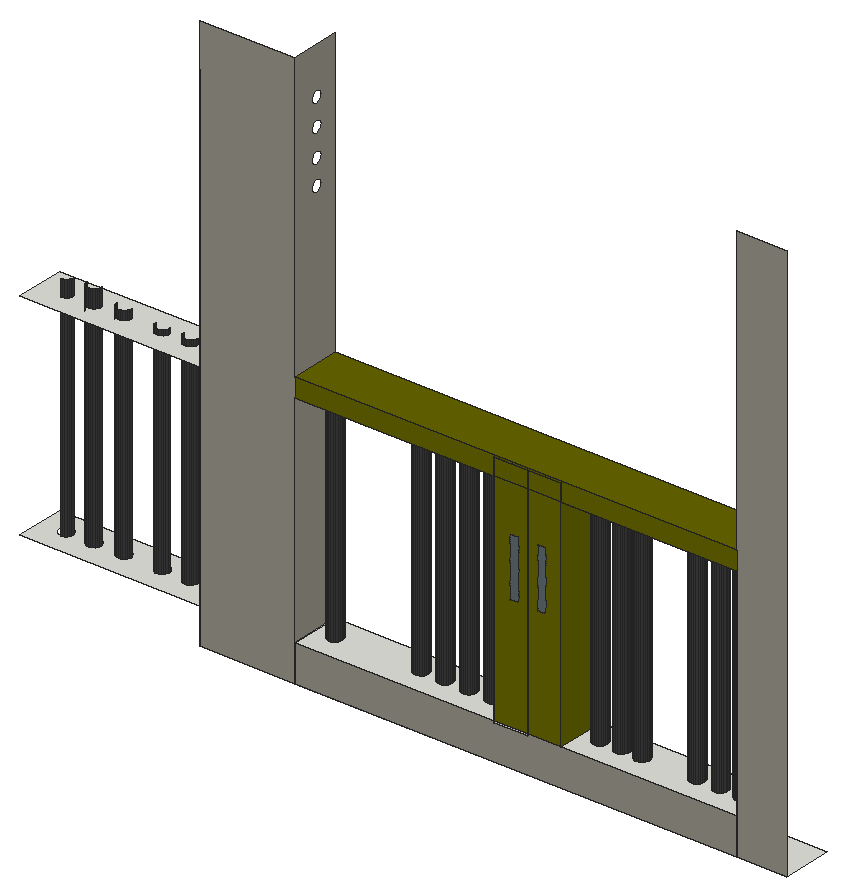
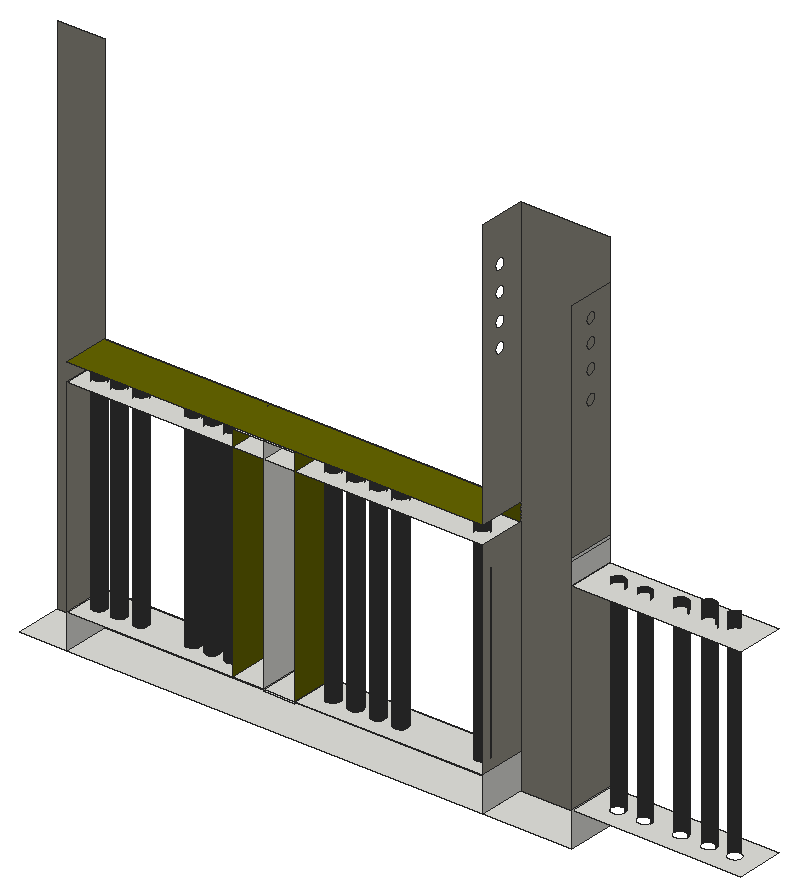
# SketchUp Ruby script. Lengths in inches.
U = 1.inch
M = Sketchup.active_model
def pt(a) = Geom::Point3d.new(a.map { |v| v * U })
def face(e, loops, mat)
  f = e.add_face(loops[0].map { |a| pt(a) })
  loops[1..].each { |l| e.add_face(l.map { |a| pt(a) }).erase! }
  f.material = f.back_material = mat if mat
  f
end
# faces: each face lists its corners as indices into pts; further lists are holes
def faces(e, pts, list, mat = nil) = list.each { |f| face(e, (f[0].is_a?(Array) ? f : [f]).map { |l| l.map { |i| pts[i] } }, mat) }
# xy, xz, yz: faces in a plane at the given z, y or x. An outline is a flat list of corners, or four numbers for a rectangle; further outlines are holes
def ring(l) = l.size == 4 ? [[l[0], l[1]], [l[2], l[1]], [l[2], l[3]], [l[0], l[3]]] : l.each_slice(2).to_a
def flat(e, list, mat, &to3) = list.each { |f| face(e, (f[0].is_a?(Array) ? f : [f]).map { |l| ring(l).map { |u, v| to3.(u, v) } }, mat) }
def xy(e, z, list, mat = nil) = flat(e, list, mat) { |x, y| [x, y, z] }
def xz(e, y, list, mat = nil) = flat(e, list, mat) { |x, z| [x, y, z] }
def yz(e, x, list, mat = nil) = flat(e, list, mat) { |y, z| [x, y, z] }
def lines(e, pts, list) = list.each { |a, b| e.add_line(pt(pts[a]), pt(pts[b])) }
# prism: a flat outline (further loops are holes) pulled along v
def prism(e, loops, v, mat = nil)
  f = face(e, loops, mat); d = Geom::Vector3d.new(v.map { |x| x * U })
  f.pushpull(f.normal.samedirection?(d) ? d.length : -d.length)
end
def box(e, o, s, mat = nil) = prism(e, [[o, [o[0] + s[0], o[1], o[2]], [o[0] + s[0], o[1] + s[1], o[2]], [o[0], o[1] + s[1], o[2]]]], [0, 0, s[2]], mat)
def at(x, y, z, deg = 0) = Geom::Transformation.translation(pt([x, y, z])) * Geom::Transformation.rotation(ORIGIN, Z_AXIS, deg.degrees)
def axes(o, x, y, z) = Geom::Transformation.new([*x, 0, *y, 0, *z, 0, *pt(o).to_a, 1])
def part(name) = M.definitions.add(name)
# library, detail: a bought-in or finely detailed component or shape, given as its bounding box
def library(name, o, s) = part(name).tap { |d| box(d.entities, o, s) }
def detail(e, o, s) = box(e.add_group.entities, o, s)
def put(e, d, t, mat = nil) = e.add_instance(d, t).tap { |i| i.material = mat if mat }
def group(e, t, mat = nil) = e.add_group.tap { |g| g.transformation = t; g.material = mat if mat }.entities
root = M.entities
M.materials.add("[Color E08]").color = [102, 102, 0]
M.materials.add("[Color M07]").color = [58, 58, 58]
M.materials.add("[Formica Graystone]").color = [149, 146, 135]
M.materials.add("[Formica Speckled Grey]").color = [94, 105, 111]
xy(root,0,[[82.62,52.46,91.56,57.16],[91.56,52.46,133.09,57.16],[133.09,52.46,137.78,57.16]])
xy(root,3.25,[[110.32,52.46,113.44,57.16]])
xy(root,3.4375,[[[65.76,52.46,82.62,57.16],[68.11,54.27,67.9375,54.29,67.77,54.36,67.63,54.47,67.52,54.61,67.45,54.78,67.43,54.96,67.45,55.13,67.52,55.3,67.63,55.44,67.77,55.55,67.9375,55.62,68.11,55.64,68.29,55.62,68.46,55.55,68.6,55.44,68.71,55.3,68.78,55.13,68.8,54.96,68.78,54.78,68.71,54.61,68.6,54.47,68.46,54.36,68.29,54.29],[79.8,54.27,79.625,54.29,79.46,54.36,79.32,54.47,79.21,54.61,79.14,54.78,79.11,54.96,79.14,55.13,79.21,55.3,79.32,55.44,79.46,55.55,79.625,55.62,79.8,55.64,79.98,55.62,80.15,55.55,80.29,55.44,80.4,55.3,80.47,55.13,80.49,54.96,80.47,54.78,80.4,54.61,80.29,54.47,80.15,54.36,79.98,54.29],[70.74,54.27,70.5625,54.29,70.4,54.36,70.25,54.47,70.14,54.61,70.07,54.78,70.05,54.96,70.07,55.13,70.14,55.3,70.25,55.44,70.4,55.55,70.5625,55.62,70.74,55.64,70.92,55.62,71.08,55.55,71.23,55.44,71.33,55.3,71.4,55.13,71.43,54.96,71.4,54.78,71.33,54.61,71.23,54.47,71.08,54.36,70.92,54.29],[77.18,54.27,77,54.29,76.83,54.36,76.69,54.47,76.58,54.61,76.51,54.78,76.49,54.96,76.51,55.13,76.58,55.3,76.69,55.44,76.83,55.55,77,55.62,77.18,55.64,77.35,55.62,77.52,55.55,77.66,55.44,77.77,55.3,77.84,55.13,77.86,54.96,77.84,54.78,77.77,54.61,77.66,54.47,77.52,54.36,77.35,54.29],[73.55,54.27,73.375,54.29,73.21,54.36,73.07,54.47,72.96,54.61,72.89,54.78,72.86,54.96,72.89,55.13,72.96,55.3,73.07,55.44,73.21,55.55,73.375,55.62,73.55,55.64,73.73,55.62,73.9,55.55,74.04,55.44,74.15,55.3,74.22,55.13,74.24,54.96,74.22,54.78,74.15,54.61,74.04,54.47,73.9,54.36,73.73,54.29]],[91.56,52.46,110.32,57.16],[110.32,52.46,113.44,57.16],[113.44,52.46,116.56,57.16],[116.56,52.46,133.09,57.16]])
xy(root,23.55,[[65.76,52.46,82.62,57.16]])
xy(root,24.05,[[91.56,52.46,133.09,57.16]])
xy(root,25.6875,[[110.32,52.46,113.44,57.16],[113.44,52.46,116.56,57.16]])
xy(root,25.83,[[91.56,52.46,133.09,57.16]],"[Color E08]")
xz(root,52.46,[[110.32,3.25,113.44,3.4375]])
xz(root,52.46,[[[110.32,3.4375,113.44,24.05],[111.77,14.14,112.58,19.7]],[[113.44,3.4375,116.56,24.05],[114.39,14.14,115.2,19.7]],[91.56,24.05,110.32,24.05,110.32,25.6875,116.56,25.6875,116.56,24.05,133.09,24.05,133.09,25.83,91.56,25.83],[110.32,24.05,113.44,25.6875],[113.44,24.05,116.56,25.6875]],"[Color E08]")
xz(root,52.46,[[82.62,0,91.56,52.6875],[91.56,0,133.09,0,133.09,3.4375,113.44,3.4375,113.44,3.25,110.32,3.25,110.32,3.4375,91.56,3.4375],[133.09,0,137.78,52.6875]],"[Formica Graystone]")
xz(root,52.46,[[111.77,14.14,112.58,19.7],[114.39,14.14,115.2,19.7]],"[Formica Speckled Grey]")
yz(root,82.62,[[52.46,0,57.16,3.4375],[52.46,23.55,57.16,25.6875],[52.46,25.6875,57.16,26.02]])
yz(root,82.62,[[52.46,3.4375,57.16,23.55],[[52.46,26.02,57.16,48.59],[54.84,38.61,54.99,38.63,55.12,38.68,55.24,38.77,55.33,38.89,55.38,39.03,55.4,39.17,55.38,39.32,55.33,39.45,55.24,39.57,55.12,39.66,54.99,39.72,54.84,39.73,54.69,39.72,54.56,39.66,54.44,39.57,54.35,39.45,54.3,39.32,54.28,39.17,54.3,39.03,54.35,38.89,54.44,38.77,54.56,38.68,54.69,38.63],[54.84,41.36,54.99,41.38,55.12,41.43,55.24,41.52,55.33,41.64,55.38,41.78,55.4,41.92,55.38,42.07,55.33,42.2,55.24,42.32,55.12,42.41,54.99,42.47,54.84,42.48,54.69,42.47,54.56,42.41,54.44,42.32,54.35,42.2,54.3,42.07,54.28,41.92,54.3,41.78,54.35,41.64,54.44,41.52,54.56,41.43,54.69,41.38],[54.84,43.67,54.99,43.69,55.12,43.75,55.24,43.84,55.33,43.95,55.38,44.09,55.4,44.23,55.38,44.38,55.33,44.52,55.24,44.63,55.12,44.72,54.99,44.78,54.84,44.8,54.69,44.78,54.56,44.72,54.44,44.63,54.35,44.52,54.3,44.38,54.28,44.23,54.3,44.09,54.35,43.95,54.44,43.84,54.56,43.75,54.69,43.69],[54.84,45.92,54.99,45.94,55.12,46,55.24,46.09,55.33,46.2,55.38,46.34,55.4,46.48,55.38,46.63,55.33,46.77,55.24,46.88,55.12,46.97,54.99,47.03,54.84,47.05,54.69,47.03,54.56,46.97,54.44,46.88,54.35,46.77,54.3,46.63,54.28,46.48,54.3,46.34,54.35,46.2,54.44,46.09,54.56,46,54.69,45.94]]],"[Formica Graystone]")
yz(root,91.56,[[52.46,0,57.16,3.4375]])
yz(root,91.56,[[52.46,3.4375,57.16,24.05],[[52.46,25.83,57.16,52.6875],[55.04,40.18,54.9,40.2,54.76,40.26,54.64,40.35,54.55,40.46,54.5,40.6,54.48,40.75,54.5,40.89,54.55,41.03,54.64,41.14,54.76,41.23,54.9,41.29,55.04,41.31,55.1875,41.29,55.32,41.23,55.4375,41.14,55.53,41.03,55.58,40.89,55.6,40.75,55.58,40.6,55.53,40.46,55.4375,40.35,55.32,40.26,55.1875,40.2],[55.04,47.68,54.9,47.7,54.76,47.76,54.64,47.85,54.55,47.96,54.5,48.1,54.48,48.25,54.5,48.39,54.55,48.53,54.64,48.64,54.76,48.73,54.9,48.79,55.04,48.81,55.1875,48.79,55.32,48.73,55.4375,48.64,55.53,48.53,55.58,48.39,55.6,48.25,55.58,48.1,55.53,47.96,55.4375,47.85,55.32,47.76,55.1875,47.7],[55.04,45.18,54.9,45.2,54.76,45.26,54.64,45.35,54.55,45.46,54.5,45.6,54.48,45.75,54.5,45.89,54.55,46.03,54.64,46.14,54.76,46.23,54.9,46.29,55.04,46.31,55.1875,46.29,55.32,46.23,55.4375,46.14,55.53,46.03,55.58,45.89,55.6,45.75,55.58,45.6,55.53,45.46,55.4375,45.35,55.32,45.26,55.1875,45.2],[55.04,42.56,54.9,42.58,54.76,42.63,54.64,42.72,54.55,42.84,54.5,42.98,54.48,43.12,54.5,43.27,54.55,43.4,54.64,43.52,54.76,43.61,54.9,43.66,55.04,43.68,55.1875,43.66,55.32,43.61,55.4375,43.52,55.53,43.4,55.58,43.27,55.6,43.12,55.58,42.98,55.53,42.84,55.4375,42.72,55.32,42.63,55.1875,42.58]]],"[Formica Graystone]")
yz(root,110.32,[[52.46,3.25,57.16,3.4375]])
yz(root,110.32,[[52.46,3.4375,57.16,25.6875]],"[Color E08]")
yz(root,113.44,[[52.46,3.25,57.16,3.4375],[52.46,3.4375,57.16,25.6875]])
yz(root,116.56,[[52.46,3.4375,57.16,25.6875]],"[Color E08]")
yz(root,133.09,[[52.46,0,57.16,3.4375]])
yz(root,133.09,[[52.46,3.4375,57.16,24.05]],"[Formica Graystone]")
p = [[68.11,54.27,3.4375],[68.29,54.29,3.4375],[68.29,54.29,25.0625],[68.11,54.27,25.0625],[68.46,54.36,3.4375],[68.46,54.36,25.0625],
  [70.4,54.36,3.4375],[70.5625,54.29,3.4375],[70.5625,54.29,25.1875],[70.4,54.36,25.1875],[70.74,54.27,3.4375],[70.74,54.27,25.1875],
  [70.92,54.29,3.4375],[70.92,54.29,25.1875],[71.08,54.36,3.4375],[71.08,54.36,25.1875],[73.21,54.36,3.4375],[73.375,54.29,3.4375],
  [73.375,54.29,24.375],[73.21,54.36,24.375],[73.55,54.27,3.4375],[73.55,54.27,24.375],[73.73,54.29,3.4375],[73.73,54.29,24.375],
  [73.9,54.36,3.4375],[73.9,54.36,24.375],[76.83,54.36,3.4375],[77,54.29,3.4375],[77,54.29,24],[76.83,54.36,24],
  [77.18,54.27,3.4375],[77.18,54.27,24],[77.35,54.29,3.4375],[77.35,54.29,24],[77.52,54.36,3.4375],[77.52,54.36,24],
  [79.46,54.36,3.4375],[79.625,54.29,3.4375],[79.625,54.29,24.0625],[79.46,54.36,24.0625],[79.8,54.27,3.4375],[79.8,54.27,24.0625],
  [79.98,54.29,3.4375],[79.98,54.29,24.0625],[80.15,54.36,3.4375],[80.15,54.36,24.0625],[93.02,54.36,3.4375],[93.1875,54.29,3.4375],
  [93.1875,54.29,25.1875],[93.02,54.36,25.1875],[93.36,54.27,3.4375],[93.36,54.27,25.1875],[93.54,54.29,3.4375],[93.54,54.29,25.1875],
  [93.71,54.36,3.4375],[93.71,54.36,25.1875],[101.15,54.36,3.4375],[101.3125,54.29,3.4375],[101.3125,54.29,25.1875],[101.15,54.36,25.1875],
  [101.49,54.27,3.4375],[101.49,54.27,25.1875],[101.67,54.29,3.4375],[101.67,54.29,25.1875],[101.83,54.36,3.4375],[101.83,54.36,25.1875],
  [103.4,54.36,3.4375],[103.5625,54.29,3.4375],[103.5625,54.29,25.1875],[103.4,54.36,25.1875],[103.74,54.27,3.4375],[103.74,54.27,25.1875],
  [103.92,54.29,3.4375],[103.92,54.29,25.1875],[104.08,54.36,3.4375],[104.08,54.36,25.1875],[105.65,54.36,3.4375],[105.8125,54.29,3.4375],
  [105.8125,54.29,25.1875],[105.65,54.36,25.1875],[105.99,54.27,3.4375],[105.99,54.27,25.1875],[106.17,54.29,3.4375],[106.17,54.29,25.1875],
  [106.33,54.36,3.4375],[106.33,54.36,25.1875],[107.9,54.36,3.4375],[108.0625,54.29,3.4375],[108.0625,54.29,25.1875],[107.9,54.36,25.1875],
  [108.24,54.27,3.4375],[108.24,54.27,25.1875],[108.42,54.29,3.4375],[108.42,54.29,25.1875],[108.58,54.36,3.4375],[108.58,54.36,25.1875],
  [117.96,54.36,3.4375],[118.125,54.29,3.4375],[118.125,54.29,25.1875],[117.96,54.36,25.1875],[118.3,54.27,3.4375],[118.3,54.27,25.1875],
  [118.48,54.29,3.4375],[118.48,54.29,25.1875],[118.65,54.36,3.4375],[118.65,54.36,25.1875],[119.96,54.36,3.4375],[120.125,54.29,3.4375],
  [120.125,54.29,25.1875],[119.96,54.36,25.1875],[120.3,54.27,3.4375],[120.3,54.27,25.1875],[120.48,54.29,3.4375],[120.48,54.29,25.1875],
  [120.65,54.36,3.4375],[120.65,54.36,25.1875],[121.9,54.36,3.4375],[122.0625,54.29,3.4375],[122.0625,54.29,25.1875],[121.9,54.36,25.1875],
  [122.24,54.27,3.4375],[122.24,54.27,25.1875],[122.42,54.29,3.4375],[122.42,54.29,25.1875],[122.58,54.36,3.4375],[122.58,54.36,25.1875],
  [127.08,54.36,3.4375],[127.25,54.29,3.4375],[127.25,54.29,25.1875],[127.08,54.36,25.1875],[127.43,54.27,3.4375],[127.43,54.27,25.1875],
  [127.6,54.29,3.4375],[127.6,54.29,25.1875],[127.77,54.36,3.4375],[127.77,54.36,25.1875],[129.27,54.36,3.4375],[129.4375,54.29,3.4375],
  [129.4375,54.29,25.1875],[129.27,54.36,25.1875],[129.61,54.27,3.4375],[129.61,54.27,25.1875],[129.79,54.29,3.4375],[129.79,54.29,25.1875],
  [129.96,54.36,3.4375],[129.96,54.36,25.1875],[131.27,54.36,3.4375],[131.4375,54.29,3.4375],[131.4375,54.29,25.1875],[131.27,54.36,25.1875],
  [131.61,54.27,3.4375],[131.61,54.27,25.1875],[131.79,54.29,3.4375],[131.79,54.29,25.1875],[131.96,54.36,3.4375],[131.96,54.36,25.1875],
  [68.6,54.47,3.4375],[68.6,54.47,25.0625],[70.25,54.47,3.4375],[70.25,54.47,25.1875],[71.23,54.47,3.4375],[71.23,54.47,25.1875],
  [73.07,54.47,3.4375],[73.07,54.47,24.375],[74.04,54.47,3.4375],[74.04,54.47,24.375],[76.69,54.47,3.4375],[76.69,54.47,24],
  [77.66,54.47,3.4375],[77.66,54.47,24],[79.32,54.47,3.4375],[79.32,54.47,24.0625],[80.29,54.47,3.4375],[80.29,54.47,24.0625],
  [92.88,54.47,3.4375],[92.88,54.47,25.1875],[93.85,54.47,3.4375],[93.85,54.47,25.1875],[101,54.47,3.4375],[101,54.47,25.1875],
  [101.98,54.47,3.4375],[101.98,54.47,25.1875],[103.25,54.47,3.4375],[103.25,54.47,25.1875],[104.23,54.47,3.4375],[104.23,54.47,25.1875],
  [105.5,54.47,3.4375],[105.5,54.47,25.1875],[106.48,54.47,3.4375],[106.48,54.47,25.1875],[107.75,54.47,3.4375],[107.75,54.47,25.1875],
  [108.73,54.47,3.4375],[108.73,54.47,25.1875],[117.82,54.47,3.4375],[117.82,54.47,25.1875],[118.79,54.47,3.4375],[118.79,54.47,25.1875],
  [119.82,54.47,3.4375],[119.82,54.47,25.1875],[120.79,54.47,3.4375],[120.79,54.47,25.1875],[121.75,54.47,3.4375],[121.75,54.47,25.1875],
  [122.73,54.47,3.4375],[122.73,54.47,25.1875],[126.94,54.47,3.4375],[126.94,54.47,25.1875],[127.91,54.47,3.4375],[127.91,54.47,25.1875],
  [129.13,54.47,3.4375],[129.13,54.47,25.1875],[130.1,54.47,3.4375],[130.1,54.47,25.1875],[131.13,54.47,3.4375],[131.13,54.47,25.1875],
  [132.1,54.47,3.4375],[132.1,54.47,25.1875],[68.71,54.61,3.4375],[68.71,54.61,25.0625],[70.14,54.61,3.4375],[70.14,54.61,25.1875],
  [71.33,54.61,3.4375],[71.33,54.61,25.1875],[72.96,54.61,3.4375],[72.96,54.61,24.375],[74.15,54.61,3.4375],[74.15,54.61,24.375],
  [76.58,54.61,3.4375],[76.58,54.61,24],[77.77,54.61,3.4375],[77.77,54.61,24],[79.21,54.61,3.4375],[79.21,54.61,24.0625],
  [80.4,54.61,3.4375],[80.4,54.61,24.0625],[92.77,54.61,3.4375],[92.77,54.61,25.1875],[93.96,54.61,3.4375],[93.96,54.61,25.1875],
  [100.89,54.61,3.4375],[100.89,54.61,25.1875],[102.08,54.61,3.4375],[102.08,54.61,25.1875],[103.14,54.61,3.4375],[103.14,54.61,25.1875],
  [104.33,54.61,3.4375],[104.33,54.61,25.1875],[105.39,54.61,3.4375],[105.39,54.61,25.1875],[106.58,54.61,3.4375],[106.58,54.61,25.1875],
  [107.64,54.61,3.4375],[107.64,54.61,25.1875],[108.83,54.61,3.4375],[108.83,54.61,25.1875],[117.71,54.61,3.4375],[117.71,54.61,25.1875],
  [118.9,54.61,3.4375],[118.9,54.61,25.1875],[119.71,54.61,3.4375],[119.71,54.61,25.1875],[120.9,54.61,3.4375],[120.9,54.61,25.1875],
  [121.64,54.61,3.4375],[121.64,54.61,25.1875],[122.83,54.61,3.4375],[122.83,54.61,25.1875],[126.83,54.61,3.4375],[126.83,54.61,25.1875],
  [128.02,54.61,3.4375],[128.02,54.61,25.1875],[129.02,54.61,3.4375],[129.02,54.61,25.1875],[130.21,54.61,3.4375],[130.21,54.61,25.1875],
  [131.02,54.61,3.4375],[131.02,54.61,25.1875],[132.21,54.61,3.4375],[132.21,54.61,25.1875],[68.78,54.78,3.4375],[68.78,54.78,25.0625],
  [70.07,54.78,3.4375],[70.07,54.78,25.1875],[71.4,54.78,3.4375],[71.4,54.78,25.1875],[72.89,54.78,3.4375],[72.89,54.78,24.375],
  [74.22,54.78,3.4375],[74.22,54.78,24.375],[76.51,54.78,3.4375],[76.51,54.78,24],[77.84,54.78,3.4375],[77.84,54.78,24],
  [79.14,54.78,3.4375],[79.14,54.78,24.0625],[80.47,54.78,3.4375],[80.47,54.78,24.0625],[92.7,54.78,3.4375],[92.7,54.78,25.1875],
  [94.03,54.78,3.4375],[94.03,54.78,25.1875],[100.82,54.78,3.4375],[100.82,54.78,25.1875],[102.15,54.78,3.4375],[102.15,54.78,25.1875],
  [103.07,54.78,3.4375],[103.07,54.78,25.1875],[104.4,54.78,3.4375],[104.4,54.78,25.1875],[105.32,54.78,3.4375],[105.32,54.78,25.1875],
  [106.65,54.78,3.4375],[106.65,54.78,25.1875],[107.57,54.78,3.4375],[107.57,54.78,25.1875],[108.9,54.78,3.4375],[108.9,54.78,25.1875],
  [117.64,54.78,3.4375],[117.64,54.78,25.1875],[118.97,54.78,3.4375],[118.97,54.78,25.1875],[119.64,54.78,3.4375],[119.64,54.78,25.1875],
  [120.97,54.78,3.4375],[120.97,54.78,25.1875],[121.57,54.78,3.4375],[121.57,54.78,25.1875],[122.9,54.78,3.4375],[122.9,54.78,25.1875],
  [126.76,54.78,3.4375],[126.76,54.78,25.1875],[128.09,54.78,3.4375],[128.09,54.78,25.1875],[128.95,54.78,3.4375],[128.95,54.78,25.1875],
  [130.28,54.78,3.4375],[130.28,54.78,25.1875],[130.95,54.78,3.4375],[130.95,54.78,25.1875],[132.28,54.78,3.4375],[132.28,54.78,25.1875],
  [68.8,54.96,3.4375],[68.8,54.96,25.0625],[70.05,54.96,3.4375],[70.05,54.96,25.1875],[71.43,54.96,3.4375],[71.43,54.96,25.1875],
  [72.86,54.96,3.4375],[72.86,54.96,24.375],[74.24,54.96,3.4375],[74.24,54.96,24.375],[76.49,54.96,3.4375],[76.49,54.96,24],
  [77.86,54.96,3.4375],[77.86,54.96,24],[79.11,54.96,3.4375],[79.11,54.96,24.0625],[80.49,54.96,3.4375],[80.49,54.96,24.0625],
  [92.68,54.96,3.4375],[92.68,54.96,25.1875],[94.05,54.96,3.4375],[94.05,54.96,25.1875],[100.8,54.96,3.4375],[100.8,54.96,25.1875],
  [102.18,54.96,3.4375],[102.18,54.96,25.1875],[103.05,54.96,3.4375],[103.05,54.96,25.1875],[104.43,54.96,3.4375],[104.43,54.96,25.1875],
  [105.3,54.96,3.4375],[105.3,54.96,25.1875],[106.68,54.96,3.4375],[106.68,54.96,25.1875],[107.55,54.96,3.4375],[107.55,54.96,25.1875],
  [108.93,54.96,3.4375],[108.93,54.96,25.1875],[117.61,54.96,3.4375],[117.61,54.96,25.1875],[118.99,54.96,3.4375],[118.99,54.96,25.1875],
  [119.61,54.96,3.4375],[119.61,54.96,25.1875],[120.99,54.96,3.4375],[120.99,54.96,25.1875],[121.55,54.96,3.4375],[121.55,54.96,25.1875],
  [122.93,54.96,3.4375],[122.93,54.96,25.1875],[126.74,54.96,3.4375],[126.74,54.96,25.1875],[128.11,54.96,3.4375],[128.11,54.96,25.1875],
  [128.93,54.96,3.4375],[128.93,54.96,25.1875],[130.3,54.96,3.4375],[130.3,54.96,25.1875],[130.93,54.96,3.4375],[130.93,54.96,25.1875],
  [132.3,54.96,3.4375],[132.3,54.96,25.1875],[92.7,55.13,3.4375],[92.7,55.13,25.1875],[94.03,55.13,3.4375],[94.03,55.13,25.1875],
  [100.82,55.13,3.4375],[100.82,55.13,25.1875],[102.15,55.13,3.4375],[102.15,55.13,25.1875],[103.07,55.13,3.4375],[103.07,55.13,25.1875],
  [104.4,55.13,3.4375],[104.4,55.13,25.1875],[105.32,55.13,3.4375],[105.32,55.13,25.1875],[106.65,55.13,3.4375],[106.65,55.13,25.1875],
  [107.57,55.13,3.4375],[107.57,55.13,25.1875],[108.9,55.13,3.4375],[108.9,55.13,25.1875],[117.64,55.13,3.4375],[117.64,55.13,25.1875],
  [118.97,55.13,3.4375],[118.97,55.13,25.1875],[119.64,55.13,3.4375],[119.64,55.13,25.1875],[120.97,55.13,3.4375],[120.97,55.13,25.1875],
  [121.57,55.13,3.4375],[121.57,55.13,25.1875],[122.9,55.13,3.4375],[122.9,55.13,25.1875],[126.76,55.13,3.4375],[126.76,55.13,25.1875],
  [128.09,55.13,3.4375],[128.09,55.13,25.1875],[128.95,55.13,3.4375],[128.95,55.13,25.1875],[130.28,55.13,3.4375],[130.28,55.13,25.1875],
  [130.95,55.13,3.4375],[130.95,55.13,25.1875],[132.28,55.13,3.4375],[132.28,55.13,25.1875],[92.77,55.3,3.4375],[92.77,55.3,25.1875],
  [93.96,55.3,3.4375],[93.96,55.3,25.1875],[100.89,55.3,3.4375],[100.89,55.3,25.1875],[102.08,55.3,3.4375],[102.08,55.3,25.1875],
  [103.14,55.3,3.4375],[103.14,55.3,25.1875],[104.33,55.3,3.4375],[104.33,55.3,25.1875],[105.39,55.3,3.4375],[105.39,55.3,25.1875],
  [106.58,55.3,3.4375],[106.58,55.3,25.1875],[107.64,55.3,3.4375],[107.64,55.3,25.1875],[108.83,55.3,3.4375],[108.83,55.3,25.1875],
  [117.71,55.3,3.4375],[117.71,55.3,25.1875],[118.9,55.3,3.4375],[118.9,55.3,25.1875],[119.71,55.3,3.4375],[119.71,55.3,25.1875],
  [120.9,55.3,3.4375],[120.9,55.3,25.1875],[121.64,55.3,3.4375],[121.64,55.3,25.1875],[122.83,55.3,3.4375],[122.83,55.3,25.1875],
  [126.83,55.3,3.4375],[126.83,55.3,25.1875],[128.02,55.3,3.4375],[128.02,55.3,25.1875],[129.02,55.3,3.4375],[129.02,55.3,25.1875],
  [130.21,55.3,3.4375],[130.21,55.3,25.1875],[131.02,55.3,3.4375],[131.02,55.3,25.1875],[132.21,55.3,3.4375],[132.21,55.3,25.1875],
  [92.88,55.44,3.4375],[92.88,55.44,25.1875],[93.85,55.44,3.4375],[93.85,55.44,25.1875],[101,55.44,3.4375],[101,55.44,25.1875],
  [101.98,55.44,3.4375],[101.98,55.44,25.1875],[103.25,55.44,3.4375],[103.25,55.44,25.1875],[104.23,55.44,3.4375],[104.23,55.44,25.1875],
  [105.5,55.44,3.4375],[105.5,55.44,25.1875],[106.48,55.44,3.4375],[106.48,55.44,25.1875],[107.75,55.44,3.4375],[107.75,55.44,25.1875],
  [108.73,55.44,3.4375],[108.73,55.44,25.1875],[117.82,55.44,3.4375],[117.82,55.44,25.1875],[118.79,55.44,3.4375],[118.79,55.44,25.1875],
  [119.82,55.44,3.4375],[119.82,55.44,25.1875],[120.79,55.44,3.4375],[120.79,55.44,25.1875],[121.75,55.44,3.4375],[121.75,55.44,25.1875],
  [122.73,55.44,3.4375],[122.73,55.44,25.1875],[126.94,55.44,3.4375],[126.94,55.44,25.1875],[127.91,55.44,3.4375],[127.91,55.44,25.1875],
  [129.13,55.44,3.4375],[129.13,55.44,25.1875],[130.1,55.44,3.4375],[130.1,55.44,25.1875],[131.13,55.44,3.4375],[131.13,55.44,25.1875],
  [132.1,55.44,3.4375],[132.1,55.44,25.1875],[93.02,55.55,3.4375],[93.02,55.55,25.1875],[93.71,55.55,3.4375],[93.71,55.55,25.1875],
  [101.15,55.55,3.4375],[101.15,55.55,25.1875],[101.83,55.55,3.4375],[101.83,55.55,25.1875],[103.4,55.55,3.4375],[103.4,55.55,25.1875],
  [104.08,55.55,3.4375],[104.08,55.55,25.1875],[105.65,55.55,3.4375],[105.65,55.55,25.1875],[106.33,55.55,3.4375],[106.33,55.55,25.1875],
  [107.9,55.55,3.4375],[107.9,55.55,25.1875],[108.58,55.55,3.4375],[108.58,55.55,25.1875],[117.96,55.55,3.4375],[117.96,55.55,25.1875],
  [118.65,55.55,3.4375],[118.65,55.55,25.1875],[119.96,55.55,3.4375],[119.96,55.55,25.1875],[120.65,55.55,3.4375],[120.65,55.55,25.1875],
  [121.9,55.55,3.4375],[121.9,55.55,25.1875],[122.58,55.55,3.4375],[122.58,55.55,25.1875],[127.08,55.55,3.4375],[127.08,55.55,25.1875],
  [127.77,55.55,3.4375],[127.77,55.55,25.1875],[129.27,55.55,3.4375],[129.27,55.55,25.1875],[129.96,55.55,3.4375],[129.96,55.55,25.1875],
  [131.27,55.55,3.4375],[131.27,55.55,25.1875],[131.96,55.55,3.4375],[131.96,55.55,25.1875],[93.1875,55.62,3.4375],[93.1875,55.62,25.1875],
  [93.36,55.64,3.4375],[93.36,55.64,25.1875],[93.54,55.62,3.4375],[93.54,55.62,25.1875],[101.3125,55.62,3.4375],[101.3125,55.62,25.1875],
  [101.49,55.64,3.4375],[101.49,55.64,25.1875],[101.67,55.62,3.4375],[101.67,55.62,25.1875],[103.5625,55.62,3.4375],[103.5625,55.62,25.1875],
  [103.74,55.64,3.4375],[103.74,55.64,25.1875],[103.92,55.62,3.4375],[103.92,55.62,25.1875],[105.8125,55.62,3.4375],[105.8125,55.62,25.1875],
  [105.99,55.64,3.4375],[105.99,55.64,25.1875],[106.17,55.62,3.4375],[106.17,55.62,25.1875],[108.0625,55.62,3.4375],[108.0625,55.62,25.1875],
  [108.24,55.64,3.4375],[108.24,55.64,25.1875],[108.42,55.62,3.4375],[108.42,55.62,25.1875],[118.125,55.62,3.4375],[118.125,55.62,25.1875],
  [118.3,55.64,3.4375],[118.3,55.64,25.1875],[118.48,55.62,3.4375],[118.48,55.62,25.1875],[120.125,55.62,3.4375],[120.125,55.62,25.1875],
  [120.3,55.64,3.4375],[120.3,55.64,25.1875],[120.48,55.62,3.4375],[120.48,55.62,25.1875],[122.0625,55.62,3.4375],[122.0625,55.62,25.1875],
  [122.24,55.64,3.4375],[122.24,55.64,25.1875],[122.42,55.62,3.4375],[122.42,55.62,25.1875],[127.25,55.62,3.4375],[127.25,55.62,25.1875],
  [127.43,55.64,3.4375],[127.43,55.64,25.1875],[127.6,55.62,3.4375],[127.6,55.62,25.1875],[129.4375,55.62,3.4375],[129.4375,55.62,25.1875],
  [129.61,55.64,3.4375],[129.61,55.64,25.1875],[129.79,55.62,3.4375],[129.79,55.62,25.1875],[131.4375,55.62,3.4375],[131.4375,55.62,25.1875],
  [131.61,55.64,3.4375],[131.61,55.64,25.1875],[131.79,55.62,3.4375],[131.79,55.62,25.1875]]
faces(root,p,[[0,1,2,3],[1,4,5,2],[6,7,8,9],[7,10,11,8],[10,12,13,11],[12,14,15,13],[16,17,18,19],[17,20,21,18],
  [20,22,23,21],[22,24,25,23],[26,27,28,29],[27,30,31,28],[30,32,33,31],[32,34,35,33],[36,37,38,39],[37,40,41,38],
  [40,42,43,41],[42,44,45,43],[46,47,48,49],[47,50,51,48],[50,52,53,51],[52,54,55,53],[56,57,58,59],[57,60,61,58],
  [60,62,63,61],[62,64,65,63],[66,67,68,69],[67,70,71,68],[70,72,73,71],[72,74,75,73],[76,77,78,79],[77,80,81,78],
  [80,82,83,81],[82,84,85,83],[86,87,88,89],[87,90,91,88],[90,92,93,91],[92,94,95,93],[96,97,98,99],[97,100,101,98],
  [100,102,103,101],[102,104,105,103],[106,107,108,109],[107,110,111,108],[110,112,113,111],[112,114,115,113],[116,117,118,119],[117,120,121,118],
  [120,122,123,121],[122,124,125,123],[126,127,128,129],[127,130,131,128],[130,132,133,131],[132,134,135,133],[136,137,138,139],[137,140,141,138],
  [140,142,143,141],[142,144,145,143],[146,147,148,149],[147,150,151,148],[150,152,153,151],[152,154,155,153],[4,156,157,5],[158,6,9,159],
  [14,160,161,15],[162,16,19,163],[24,164,165,25],[166,26,29,167],[34,168,169,35],[170,36,39,171],[44,172,173,45],[174,46,49,175],
  [54,176,177,55],[178,56,59,179],[64,180,181,65],[182,66,69,183],[74,184,185,75],[186,76,79,187],[84,188,189,85],[190,86,89,191],
  [94,192,193,95],[194,96,99,195],[104,196,197,105],[198,106,109,199],[114,200,201,115],[202,116,119,203],[124,204,205,125],[206,126,129,207],
  [134,208,209,135],[210,136,139,211],[144,212,213,145],[214,146,149,215],[154,216,217,155],[156,218,219,157],[220,158,159,221],[160,222,223,161],
  [224,162,163,225],[164,226,227,165],[228,166,167,229],[168,230,231,169],[232,170,171,233],[172,234,235,173],[236,174,175,237],[176,238,239,177],
  [240,178,179,241],[180,242,243,181],[244,182,183,245],[184,246,247,185],[248,186,187,249],[188,250,251,189],[252,190,191,253],[192,254,255,193],
  [256,194,195,257],[196,258,259,197],[260,198,199,261],[200,262,263,201],[264,202,203,265],[204,266,267,205],[268,206,207,269],[208,270,271,209],
  [272,210,211,273],[212,274,275,213],[276,214,215,277],[216,278,279,217],[218,280,281,219],[282,220,221,283],[222,284,285,223],[286,224,225,287],
  [226,288,289,227],[290,228,229,291],[230,292,293,231],[294,232,233,295],[234,296,297,235],[298,236,237,299],[238,300,301,239],[302,240,241,303],
  [242,304,305,243],[306,244,245,307],[246,308,309,247],[310,248,249,311],[250,312,313,251],[314,252,253,315],[254,316,317,255],[318,256,257,319],
  [258,320,321,259],[322,260,261,323],[262,324,325,263],[326,264,265,327],[266,328,329,267],[330,268,269,331],[270,332,333,271],[334,272,273,335],
  [274,336,337,275],[338,276,277,339],[278,340,341,279],[280,342,343,281],[344,282,283,345],[284,346,347,285],[348,286,287,349],[288,350,351,289],
  [352,290,291,353],[292,354,355,293],[356,294,295,357],[296,358,359,297],[360,298,299,361],[300,362,363,301],[364,302,303,365],[304,366,367,305],
  [368,306,307,369],[308,370,371,309],[372,310,311,373],[312,374,375,313],[376,314,315,377],[316,378,379,317],[380,318,319,381],[320,382,383,321],
  [384,322,323,385],[324,386,387,325],[388,326,327,389],[328,390,391,329],[392,330,331,393],[332,394,395,333],[396,334,335,397],[336,398,399,337],
  [400,338,339,401],[340,402,403,341],[404,360,361,405],[362,406,407,363],[408,364,365,409],[366,410,411,367],[412,368,369,413],[370,414,415,371],
  [416,372,373,417],[374,418,419,375],[420,376,377,421],[378,422,423,379],[424,380,381,425],[382,426,427,383],[428,384,385,429],[386,430,431,387],
  [432,388,389,433],[390,434,435,391],[436,392,393,437],[394,438,439,395],[440,396,397,441],[398,442,443,399],[444,400,401,445],[402,446,447,403],
  [448,404,405,449],[406,450,451,407],[452,408,409,453],[410,454,455,411],[456,412,413,457],[414,458,459,415],[460,416,417,461],[418,462,463,419],
  [464,420,421,465],[422,466,467,423],[468,424,425,469],[426,470,471,427],[472,428,429,473],[430,474,475,431],[476,432,433,477],[434,478,479,435],
  [480,436,437,481],[438,482,483,439],[484,440,441,485],[442,486,487,443],[488,444,445,489],[446,490,491,447],[492,448,449,493],[450,494,495,451],
  [496,452,453,497],[454,498,499,455],[500,456,457,501],[458,502,503,459],[504,460,461,505],[462,506,507,463],[508,464,465,509],[466,510,511,467],
  [512,468,469,513],[470,514,515,471],[516,472,473,517],[474,518,519,475],[520,476,477,521],[478,522,523,479],[524,480,481,525],[482,526,527,483],
  [528,484,485,529],[486,530,531,487],[532,488,489,533],[490,534,535,491],[536,492,493,537],[494,538,539,495],[540,496,497,541],[498,542,543,499],
  [544,500,501,545],[502,546,547,503],[548,504,505,549],[506,550,551,507],[552,508,509,553],[510,554,555,511],[556,512,513,557],[514,558,559,515],
  [560,516,517,561],[518,562,563,519],[564,520,521,565],[522,566,567,523],[568,524,525,569],[526,570,571,527],[572,528,529,573],[530,574,575,531],
  [576,532,533,577],[534,578,579,535],[580,536,537,581],[582,580,581,583],[584,582,583,585],[538,584,585,539],[586,540,541,587],[588,586,587,589],
  [590,588,589,591],[542,590,591,543],[592,544,545,593],[594,592,593,595],[596,594,595,597],[546,596,597,547],[598,548,549,599],[600,598,599,601],
  [602,600,601,603],[550,602,603,551],[604,552,553,605],[606,604,605,607],[608,606,607,609],[554,608,609,555],[610,556,557,611],[612,610,611,613],
  [614,612,613,615],[558,614,615,559],[616,560,561,617],[618,616,617,619],[620,618,619,621],[562,620,621,563],[622,564,565,623],[624,622,623,625],
  [626,624,625,627],[566,626,627,567],[628,568,569,629],[630,628,629,631],[632,630,631,633],[570,632,633,571],[634,572,573,635],[636,634,635,637],
  [638,636,637,639],[574,638,639,575],[640,576,577,641],[642,640,641,643],[644,642,643,645],[578,644,645,579]],"[Color M07]")
